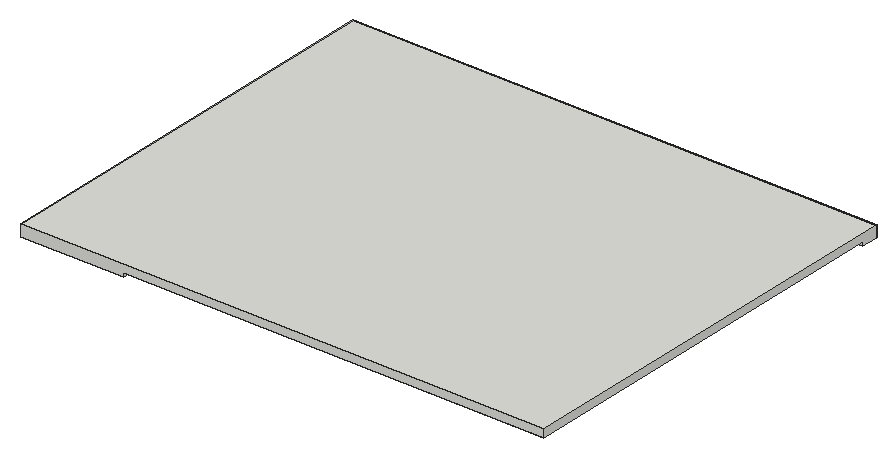
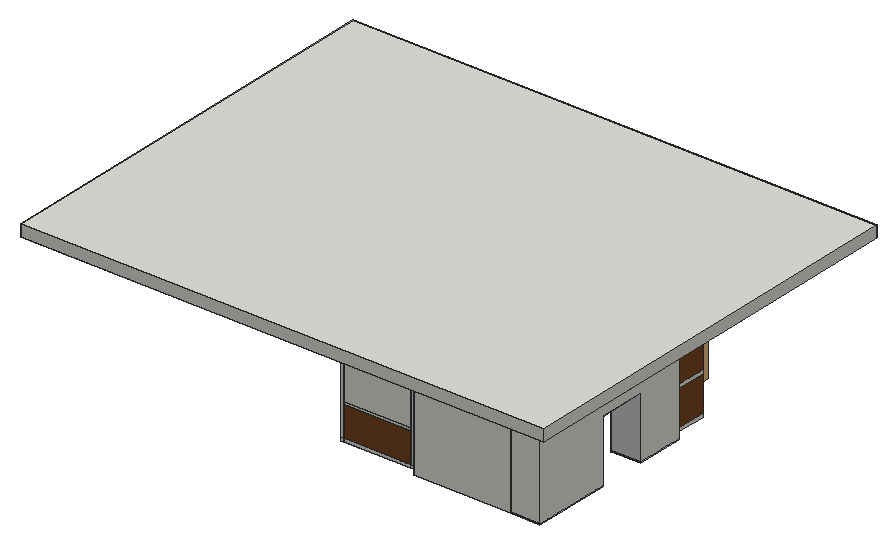
# SketchUp Ruby script. Lengths in inches.
U = 1.inch
M = Sketchup.active_model
def pt(a) = Geom::Point3d.new(a.map { |v| v * U })
def face(e, loops, mat)
  f = e.add_face(loops[0].map { |a| pt(a) })
  loops[1..].each { |l| e.add_face(l.map { |a| pt(a) }).erase! }
  f.material = f.back_material = mat if mat
  f
end
# faces: each face lists its corners as indices into pts; further lists are holes
def faces(e, pts, list, mat = nil) = list.each { |f| face(e, (f[0].is_a?(Array) ? f : [f]).map { |l| l.map { |i| pts[i] } }, mat) }
# xy, xz, yz: faces in a plane at the given z, y or x. An outline is a flat list of corners, or four numbers for a rectangle; further outlines are holes
def ring(l) = l.size == 4 ? [[l[0], l[1]], [l[2], l[1]], [l[2], l[3]], [l[0], l[3]]] : l.each_slice(2).to_a
def flat(e, list, mat, &to3) = list.each { |f| face(e, (f[0].is_a?(Array) ? f : [f]).map { |l| ring(l).map { |u, v| to3.(u, v) } }, mat) }
def xy(e, z, list, mat = nil) = flat(e, list, mat) { |x, y| [x, y, z] }
def xz(e, y, list, mat = nil) = flat(e, list, mat) { |x, z| [x, y, z] }
def yz(e, x, list, mat = nil) = flat(e, list, mat) { |y, z| [x, y, z] }
def lines(e, pts, list) = list.each { |a, b| e.add_line(pt(pts[a]), pt(pts[b])) }
# prism: a flat outline (further loops are holes) pulled along v
def prism(e, loops, v, mat = nil)
  f = face(e, loops, mat); d = Geom::Vector3d.new(v.map { |x| x * U })
  f.pushpull(f.normal.samedirection?(d) ? d.length : -d.length)
end
def box(e, o, s, mat = nil) = prism(e, [[o, [o[0] + s[0], o[1], o[2]], [o[0] + s[0], o[1] + s[1], o[2]], [o[0], o[1] + s[1], o[2]]]], [0, 0, s[2]], mat)
def at(x, y, z, deg = 0) = Geom::Transformation.translation(pt([x, y, z])) * Geom::Transformation.rotation(ORIGIN, Z_AXIS, deg.degrees)
def axes(o, x, y, z) = Geom::Transformation.new([*x, 0, *y, 0, *z, 0, *pt(o).to_a, 1])
def part(name) = M.definitions.add(name)
# library, detail: a bought-in or finely detailed component or shape, given as its bounding box
def library(name, o, s) = part(name).tap { |d| box(d.entities, o, s) }
def detail(e, o, s) = box(e.add_group.entities, o, s)
def put(e, d, t, mat = nil) = e.add_instance(d, t).tap { |i| i.material = mat if mat }
def group(e, t, mat = nil) = e.add_group.tap { |g| g.transformation = t; g.material = mat if mat }.entities
root = M.entities
M.materials.add("Emissive").color = [223, 228, 179]
M.materials.add("Generic").color = [71, 77, 71]
M.materials.add("Generic\#1").color = [198, 203, 199]
M.materials.add("Gold 10k").color = [251, 232, 180]
M.materials.add("[Wood Floor Light]").color = [204, 176, 127]
M.materials.add("[Wood Veneer 01]").color = [120, 70, 37]
c1 = library("kitchen utensils",[-21.58,227.67,74.34],[25.67,8.97,31.25])
c2 = library("Tlon Light 1950 Ceiling 152 010",[-38.39,-38.39,-3.78],[76.78,76.78,3.41])
c3 = library("Microwave 116-11",[-7.27,-5.23,0],[14.54,10.46,7.87])
c4 = library("Potted Plant 50-23",[-3.4,-3.5,0],[6.8,7,9.93])
c5 = library("Pendant 02 114-03",[-6.79,-6.8,-58.42],[13.6,13.6,58.44])
c6 = library("Peperomia 450 001",[-6.6875,-10.1875,-9.42],[16.7,12.74,19.03])
xy(root,72.9375,[[9,120.99,24.25,146.7],[9,172.41,24.25,172.41,24.25,198.875,25,198.875,25,214.125,9,214.125],[25,198.875,76.5,214.125]])
xy(root,72.9375,[[24.25,120.99,25,146.7],[24.25,172.41,25,198.125],[24.25,198.125,76.5,198.875]],"Gold 10k")
xy(root,73.34,[[9,120.99,24.25,146.7],[9,172.41,24.25,172.41,24.25,198.875,25,198.875,25,214.125,9,214.125]])
xy(root,73.34,[[24.25,120.99,25,133.84],[24.25,134.24,25,146.7],[24.25,172.41,25,185.27],[24.25,185.67,25,198.125],[24.25,198.125,25,198.875],
  [25,198.125,42.17,198.875],[42.57,198.125,59.33,198.875],[59.73,198.125,76.5,198.875]],"Gold 10k")
xy(root,74.34,[[43.57,198.125,58.33,210.125],[60.73,198.125,75.5,210.125]],"[Wood Floor Light]")
xy(root,75.04,[[10.8125,103.125,10.8125,119.26,25,119.26,25,107.5625,24.96,106.98,24.85,106.41,24.66,105.86,24.41,105.34,24.08,104.86,23.7,104.42,23.26,104.04,22.78,103.72,22.26,103.46,21.71,103.28,21.14,103.16,20.5625,103.125]],"[Wood Veneer 01]")
xy(root,75.875,[[78.25,188.8125,114.125,214.125]],"[Wood Veneer 01]")
xy(root,76.74,[[10.8125,103.125,20.5625,103.125,21.14,103.16,21.71,103.28,22.26,103.46,22.78,103.72,23.26,104.04,23.7,104.42,24.08,104.86,24.41,105.34,24.66,105.86,24.85,106.41,24.96,106.98,25,107.5625,25,119.26,10.8125,119.26]],"[Wood Veneer 01]")
xy(root,77.5,[[78.25,188.8125,114.125,214.125]],"[Wood Veneer 01]")
xy(root,85.24,[[43.57,208.125,58.33,210.125],[60.73,208.125,75.5,210.125]],"Emissive")
xy(root,85.24,[[43.57,198.3125,58.33,208.125],[60.73,198.3125,75.5,208.125]],"[Wood Floor Light]")
xy(root,86.49,[[43.57,198.3125,58.33,210.125],[60.73,198.3125,75.5,210.125]],"[Wood Floor Light]")
xy(root,93.85,[[78.25,212.125,114.125,214.125]],"Emissive")
xy(root,93.85,[[78.25,188.8125,114.125,212.125]],"[Wood Veneer 01]")
xy(root,94.92,[[78.25,188.8125,114.125,189.5625]],"Gold 10k")
xy(root,95.32,[[78.65,188.8125,95.79,189.5625],[96.1875,188.8125,113.73,189.5625]],"Gold 10k")
xy(root,96.04,[[10.8125,103.125,10.8125,119.26,25,119.26,25,107.5625,24.96,106.98,24.85,106.41,24.66,105.86,24.41,105.34,24.08,104.86,23.7,104.42,23.26,104.04,22.78,103.72,22.26,103.46,21.71,103.28,21.14,103.16,20.5625,103.125]],"[Wood Veneer 01]")
xy(root,96.68,[[43.57,208.125,58.33,210.125],[60.73,208.125,75.5,210.125]],"Emissive")
xy(root,96.68,[[43.57,198.3125,58.33,208.125],[60.73,198.3125,75.5,208.125]],"[Wood Floor Light]")
xy(root,97.74,[[10.8125,103.125,20.5625,103.125,21.14,103.16,21.71,103.28,22.26,103.46,22.78,103.72,23.26,104.04,23.7,104.42,24.08,104.86,24.41,105.34,24.66,105.86,24.85,106.41,24.96,106.98,25,107.5625,25,119.26,10.8125,119.26]],"[Wood Veneer 01]")
xy(root,97.93,[[43.57,198.3125,58.33,210.125],[60.73,198.3125,75.5,210.125]],"[Wood Floor Light]")
xy(root,106.4375,[[9,146.7,25,172.41]],"[Wood Veneer 01]")
xy(root,106.8125,[[9,146.7,24.25,172.41]])
xy(root,106.8125,[[24.25,146.7,25,172.41]],"Gold 10k")
xy(root,107.21,[[24.25,146.7,25,159.56],[24.25,159.96,25,172.41]],"Gold 10k")
xy(root,108.03,[[43.57,208.125,58.33,210.125],[60.73,208.125,75.5,210.125]],"Emissive")
xy(root,108.03,[[43.57,198.125,58.33,208.125],[60.73,198.125,75.5,208.125]],"[Wood Floor Light]")
xy(root,109.03,[[42.57,198.125,59.33,198.875],[59.73,198.125,76.5,198.875]],"Gold 10k")
xy(root,109.43,[[42.57,198.125,59.33,198.875],[59.73,198.125,76.5,198.875]],"Gold 10k")
xy(root,114.48,[[10.8125,119.26,13.21,119.92]])
xy(root,114.48,[[13.21,103.125,13.21,119.26,25,119.26,25,120.99,55.3125,120.99,55.3125,103.125]],"[Wood Veneer 01]")
xy(root,118.1,[[78.65,188.8125,95.79,189.5625],[96.1875,188.8125,113.73,189.5625]],"Gold 10k")
xy(root,118.5,[[114.125,188.8125,115.875,214.125],[78.25,189.5625,114.125,214.125]])
xy(root,118.5,[[78.25,188.8125,114.125,189.5625]],"Gold 10k")
xy(root,119.1875,[[9,120.99,9,214.125,25,214.125,25,198.125,24.25,198.125,24.25,120.99],[24.25,172.41,25,185.27],[42.57,198.125,59.33,198.875],[59.73,198.125,76.5,198.875],[25,198.875,76.5,214.125]])
xy(root,119.1875,[[24.25,120.99,25,133.84],[24.25,134.24,25,146.7],[24.25,146.7,25,159.56],[24.25,159.96,25,172.41],[24.25,185.67,25,198.125],
  [25,198.125,42.17,198.875]],"Gold 10k")
xy(root,119.4375,[[9,120.99,9,214.125,25,214.125,25,198.125,24.25,198.125,24.25,120.99],[25,198.875,76.5,214.125]])
xy(root,119.4375,[[24.25,120.99,25,198.125],[25,198.125,76.5,198.875]],"Gold 10k")
xy(root,120,[[0,0,9,223.125],[9,0,55.3125,103.125],[9,103.125,55.3125,120.99],[9,120.99,25,214.125],[76.5,188.8125,78.25,214.125],
  [78.25,188.8125,114.125,190.125],[114.125,188.8125,115.875,214.125],[78.25,190.125,114.125,214.125],[78.25,190.125,114.125,214.125],[25,198.125,76.5,214.125],
  [9,214.125,280.625,223.125]])
xy(root,120,[[[55.3125,103.125,55.3125,120.99,25,120.99,25,198.125,76.5,198.125,76.5,188.8125,115.875,188.8125,115.875,214.125,120,214.125,120,103.125],[62.86,110.67,112.45,110.67,112.45,181.27,68.95,181.27,68.95,190.58,32.55,190.58,32.55,128.53,62.86,128.53]],[48.41,135.56,48.41,176.5,55.1,176.5,55.1,140.62,103.28,140.62,103.28,135.56],[[64.44,146.92,76.63,163.8],[68.11,152.46,72.97,158.13]]],"[Wood Veneer 01]")
xy(root,122,[[55.3125,0,280.625,103.125],[[55.3125,103.125,120,103.125,120,214.125,115.875,214.125,115.875,188.8125,76.5,188.8125,76.5,198.125,25,198.125,25,120.99,55.3125,120.99],[60.86,108.67,60.86,126.53,30.55,126.53,30.55,192.58,70.95,192.58,70.95,183.27,114.45,183.27,114.45,108.67]],[120,103.125,280.625,214.125],[50.41,137.56,103.28,137.56,103.28,138.62,53.1,138.62,53.1,176.5,50.41,176.5],[[64.44,148.92,74.63,161.8],[66.11,150.46,72.97,158.13]]])
xy(root,122,[[60.86,108.67,62.86,128.53],[62.86,108.67,112.45,110.67],[112.45,108.67,114.45,181.27],[30.55,126.53,32.55,190.58],[32.55,126.53,60.86,128.53],
  [48.41,135.56,50.41,176.5],[50.41,135.56,55.1,137.56],[55.1,135.56,103.28,137.56],[53.1,138.62,55.1,176.5],[55.1,138.62,103.28,140.62],
  [64.44,146.92,74.63,148.92],[74.63,146.92,76.63,163.8],[66.11,150.46,72.97,152.46],[66.11,152.46,68.11,158.13],[64.44,161.8,74.63,163.8],
  [68.95,181.27,78.25,183.27],[78.25,181.27,114.45,183.27],[68.95,183.27,70.95,190.58],[30.55,190.58,70.95,192.58]],"Emissive")
xy(root,124,[[[60.86,108.67,60.86,126.53,30.55,126.53,30.55,192.58,70.95,192.58,70.95,183.27,114.45,183.27,114.45,108.67],[50.41,137.56,103.28,137.56,103.28,138.62,53.1,138.62,53.1,176.5,50.41,176.5],[64.44,148.92,74.63,161.8]],[66.11,150.46,72.97,158.13]])
xy(root,126,[[0,0,280.625,223.125]])
xz(root,0,[[0,120,55.3125,120,55.3125,122,280.625,122,280.625,126,0,126]])
xz(root,103.125,[[55.3125,120,120,122]])
xz(root,103.125,[[10.8125,75.04,20.5625,76.74],[10.8125,96.04,20.5625,97.74]],"[Wood Veneer 01]")
xz(root,108.67,[[60.86,122,114.45,124]],"Emissive")
xz(root,110.67,[[62.86,120,112.45,122]])
xz(root,119.26,[[10.8125,75.04,25,76.74],[10.8125,96.04,25,97.74]])
xz(root,119.26,[[10.8125,76.74,25,96.04],[10.8125,97.74,25,114.48]],"[Wood Veneer 01]")
xz(root,119.92,[[10.8125,112.09,10.8125,114.48,13.21,114.48,12.89,114.46,12.59,114.4,12.29,114.3,12.01,114.16,11.75,113.99,11.51,113.78,11.31,113.55,11.13,113.29,10.99,113,10.89,112.71,10.83,112.4]])
xz(root,120.99,[[9,72.9375,24.25,73.34],[24.25,72.9375,25,73.34],[9,73.34,25,119.1875],[9,119.1875,24.25,119.4375],[9,119.4375,25,120],
  [25,120,55.3125,122]])
xz(root,120.99,[[25,114.48,25,119.1875,24.25,119.1875,24.25,119.4375,25,119.4375,25,120,55.3125,120,55.3125,114.48]],"[Wood Veneer 01]")
xz(root,126.53,[[30.55,122,60.86,124]],"Emissive")
xz(root,128.53,[[32.55,120,62.86,122]],"[Wood Veneer 01]")
xz(root,133.84,[[24.25,73.34,25,119.1875]],"Gold 10k")
xz(root,134.24,[[24.25,73.34,25,119.1875]],"Gold 10k")
xz(root,135.56,[[48.41,120,55.1,122],[55.1,120,103.28,122]],"[Wood Veneer 01]")
xz(root,137.56,[[50.41,122,55.1,124],[55.1,122,103.28,124]],"Emissive")
xz(root,138.62,[[53.1,122,103.28,124]],"Emissive")
xz(root,140.62,[[55.1,120,103.28,122]],"[Wood Veneer 01]")
xz(root,146.7,[[9,72.9375,24.25,73.34],[9,106.4375,25,106.8125],[24.25,106.8125,25,107.21]])
xz(root,146.7,[[9,73.34,25,106.4375]],"Generic\#1")
xz(root,146.92,[[64.44,120,76.63,122]],"[Wood Veneer 01]")
xz(root,148.92,[[64.44,122,74.63,124]],"Emissive")
xz(root,150.46,[[66.11,122,72.97,124]],"Emissive")
xz(root,152.46,[[68.11,120,72.97,122]])
xz(root,158.13,[[68.11,120,72.97,122]])
xz(root,158.13,[[66.11,122,72.97,124]],"Emissive")
xz(root,159.56,[[24.25,107.21,25,119.1875]],"Gold 10k")
xz(root,159.96,[[24.25,107.21,25,119.1875]],"Gold 10k")
xz(root,161.8,[[64.44,122,74.63,124]],"Emissive")
xz(root,163.8,[[64.44,120,76.63,122]])
xz(root,172.41,[[9,106.4375,25,106.8125],[24.25,106.8125,25,107.21]])
xz(root,172.41,[[9,72.9375,24.25,73.34]],"Generic\#1")
xz(root,172.41,[[9,73.34,25,106.4375]],"[Wood Veneer 01]")
xz(root,176.5,[[48.41,120,55.1,122],[50.41,122,53.1,124]])
xz(root,181.27,[[68.95,120,78.25,122],[78.25,120,112.45,122]],"[Wood Veneer 01]")
xz(root,183.27,[[70.95,122,78.25,124],[78.25,122,114.45,124]],"Emissive")
xz(root,185.27,[[24.25,73.34,25,119.1875]],"Gold 10k")
xz(root,185.67,[[24.25,73.34,25,119.1875]],"Gold 10k")
xz(root,188.8125,[[76.5,120,78.25,122],[78.25,120,114.125,122],[114.125,120,115.875,122]])
xz(root,188.8125,[[78.65,95.32,95.79,118.1],[96.1875,95.32,113.73,118.1]],"Generic\#1")
xz(root,188.8125,[[78.25,75.875,114.125,77.5],[78.25,93.85,114.125,94.92],[78.25,118.5,114.125,120],[114.125,118.5,115.875,120]],"[Wood Veneer 01]")
xz(root,189.5625,[[[78.25,94.92,114.125,118.5],[78.65,95.32,113.73,118.1]],[95.79,95.32,96.1875,118.1]],"Gold 10k")
xz(root,190.58,[[32.55,120,68.95,122]],"[Wood Veneer 01]")
xz(root,192.58,[[30.55,122,70.95,124]],"Emissive")
xz(root,198.125,[[25,120,76.5,122]])
xz(root,198.125,[[25,73.34,42.17,119.1875]],"Generic")
xz(root,198.125,[[42.57,109.43,59.33,119.1875],[59.73,109.43,76.5,119.1875],[25,119.4375,76.5,120]],"Generic\#1")
xz(root,198.125,[[24.25,119.1875,25,119.4375]],"Gold 10k")
xz(root,198.125,[[[42.57,73.34,59.33,109.03],[43.57,74.34,58.33,108.03]],[[59.73,73.34,76.5,109.03],[60.73,74.34,75.5,108.03]]],"[Wood Floor Light]")
xz(root,198.3125,[[43.57,85.24,58.33,86.49],[60.73,85.24,75.5,86.49],[43.57,96.68,58.33,97.93],[60.73,96.68,75.5,97.93]],"[Wood Floor Light]")
xz(root,198.875,[[24.25,72.9375,25,73.34],[25,72.9375,76.5,73.34],[42.17,73.34,42.57,119.1875],[59.33,73.34,59.73,119.1875],[42.57,109.03,59.33,109.43],
  [59.73,109.03,76.5,109.43],[25,119.1875,76.5,119.4375]],"Gold 10k")
xz(root,210.125,[[43.57,85.24,58.33,86.49],[60.73,85.24,75.5,86.49],[43.57,96.68,58.33,97.93],[60.73,96.68,75.5,97.93]])
xz(root,210.125,[[43.57,74.34,58.33,85.24],[60.73,74.34,75.5,85.24],[43.57,86.49,58.33,96.68],[60.73,86.49,75.5,96.68],[43.57,97.93,58.33,108.03],
  [60.73,97.93,75.5,108.03]],"[Wood Floor Light]")
xz(root,214.125,[[9,72.9375,25,73.34],[25,72.9375,76.5,119.1875],[9,73.34,25,119.1875],[76.5,75.875,78.25,77.5],[78.25,75.875,114.125,77.5],
  [114.125,75.875,115.875,77.5],[76.5,77.5,78.25,120],[114.125,77.5,115.875,118.5],[78.25,93.85,114.125,94.92],[78.25,94.92,114.125,118.5],
  [78.25,118.5,114.125,120],[114.125,118.5,115.875,120],[9,119.1875,25,119.4375],[25,119.1875,76.5,119.4375],[9,119.4375,25,120],
  [25,119.4375,76.5,120],[115.875,120,120,122],[120,120,280.625,122]])
xz(root,214.125,[[78.25,77.5,114.125,93.85]],"[Wood Veneer 01]")
xz(root,223.125,[[0,120,280.625,126]])
yz(root,0,[[0,120,223.125,126]])
yz(root,9,[[120.99,72.9375,146.7,73.34],[172.41,72.9375,214.125,73.34],[120.99,73.34,120.99,119.1875,214.125,119.1875,214.125,73.34,172.41,73.34,172.41,106.8125,146.7,106.8125,146.7,73.34],[146.7,106.4375,172.41,106.8125],[120.99,119.1875,214.125,119.4375],
  [120.99,119.4375,214.125,120]])
yz(root,10.8125,[[103.125,75.04,119.26,76.74],[103.125,96.04,119.26,97.74],[119.26,112.09,119.92,114.48]])
yz(root,10.8125,[[103.125,76.74,119.26,96.04],[103.125,97.74,119.26,112.09]],"[Wood Veneer 01]")
yz(root,24.25,[[120.99,72.9375,146.7,73.34],[172.41,72.9375,198.875,73.34],[133.84,73.34,134.24,119.1875],[185.27,73.34,185.67,119.1875],[146.7,106.8125,172.41,107.21],
  [159.56,107.21,159.96,119.1875],[120.99,119.1875,198.125,119.4375]],"Gold 10k")
yz(root,25,[[198.875,72.9375,214.125,73.34],[198.125,73.34,214.125,119.1875],[146.7,106.4375,172.41,106.8125],[198.875,119.1875,214.125,119.4375],[198.125,119.4375,214.125,120],
  [120.99,120,198.125,122]])
yz(root,25,[[146.7,107.21,159.56,119.1875],[159.96,107.21,172.41,119.1875]],"Generic")
yz(root,25,[[120.99,73.34,133.84,119.1875],[134.24,73.34,146.7,119.1875],[172.41,73.34,185.27,119.1875],[185.67,73.34,198.125,119.1875],[120.99,119.4375,198.125,120]],"Generic\#1")
yz(root,25,[[198.125,119.1875,198.875,119.4375]],"Gold 10k")
yz(root,25,[[107.5625,75.04,119.26,76.74],[107.5625,96.04,119.26,97.74]],"[Wood Veneer 01]")
yz(root,30.55,[[126.53,122,192.58,124]],"Emissive")
yz(root,32.55,[[128.53,120,190.58,122]],"[Wood Veneer 01]")
yz(root,42.17,[[198.125,73.34,198.875,119.1875]],"Gold 10k")
yz(root,42.57,[[198.125,109.43,198.875,119.1875]])
yz(root,42.57,[[198.125,73.34,198.875,109.03]],"Gold 10k")
yz(root,43.57,[[198.3125,85.24,210.125,86.49],[198.3125,96.68,210.125,97.93]])
yz(root,43.57,[[198.125,74.34,210.125,74.34,210.125,85.24,198.3125,85.24,198.3125,86.49,210.125,86.49,210.125,96.68,198.3125,96.68,198.3125,97.93,210.125,97.93,210.125,108.03,198.125,108.03]],"[Wood Floor Light]")
yz(root,48.41,[[135.56,120,176.5,122]])
yz(root,50.41,[[137.56,122,176.5,124]],"Emissive")
yz(root,53.1,[[138.62,122,176.5,124]],"Emissive")
yz(root,55.1,[[140.62,120,176.5,122]],"[Wood Veneer 01]")
yz(root,55.3125,[[0,120,103.125,122],[103.125,120,120.99,122]])
yz(root,55.3125,[[103.125,114.48,120.99,120]],"[Wood Veneer 01]")
yz(root,58.33,[[198.3125,85.24,210.125,86.49],[198.3125,96.68,210.125,97.93]])
yz(root,58.33,[[198.125,74.34,198.125,108.03,210.125,108.03,210.125,97.93,198.3125,97.93,198.3125,96.68,210.125,96.68,210.125,86.49,198.3125,86.49,198.3125,85.24,210.125,85.24,210.125,74.34]],"[Wood Floor Light]")
yz(root,59.33,[[198.125,73.34,198.875,109.03],[198.125,109.43,198.875,119.1875]],"Gold 10k")
yz(root,59.73,[[198.125,73.34,198.875,109.03],[198.125,109.43,198.875,119.1875]],"Gold 10k")
yz(root,60.73,[[198.3125,85.24,210.125,86.49],[198.3125,96.68,210.125,97.93]])
yz(root,60.73,[[198.125,74.34,210.125,74.34,210.125,85.24,198.3125,85.24,198.3125,86.49,210.125,86.49,210.125,96.68,198.3125,96.68,198.3125,97.93,210.125,97.93,210.125,108.03,198.125,108.03]],"[Wood Floor Light]")
yz(root,60.86,[[108.67,122,126.53,124]],"Emissive")
yz(root,62.86,[[110.67,120,128.53,122]],"[Wood Veneer 01]")
yz(root,64.44,[[146.92,120,163.8,122]])
yz(root,64.44,[[148.92,122,161.8,124]],"Emissive")
yz(root,66.11,[[150.46,122,158.13,124]],"Emissive")
yz(root,68.11,[[152.46,120,158.13,122]])
yz(root,68.95,[[181.27,120,190.58,122]])
yz(root,70.95,[[183.27,122,192.58,124]],"Emissive")
yz(root,72.97,[[152.46,120,158.13,122]])
yz(root,72.97,[[150.46,122,158.13,124]],"Emissive")
yz(root,74.63,[[148.92,122,161.8,124]],"Emissive")
yz(root,75.5,[[198.3125,85.24,210.125,86.49],[198.3125,96.68,210.125,97.93]])
yz(root,75.5,[[198.125,74.34,198.125,108.03,210.125,108.03,210.125,97.93,198.3125,97.93,198.3125,96.68,210.125,96.68,210.125,86.49,198.3125,86.49,198.3125,85.24,210.125,85.24,210.125,74.34]],"[Wood Floor Light]")
yz(root,76.5,[[198.875,72.9375,214.125,72.9375,214.125,75.875,198.125,75.875,198.125,73.34,198.875,73.34],[198.125,75.875,214.125,77.5],[198.125,77.5,214.125,77.5,214.125,119.1875,198.125,119.1875,198.125,109.43,198.875,109.43,198.875,109.03,198.125,109.03],[198.875,119.1875,214.125,119.4375],[198.125,119.4375,214.125,120],
  [188.8125,120,198.125,122]])
yz(root,76.63,[[146.92,120,163.8,122]],"[Wood Veneer 01]")
yz(root,78.25,[[188.8125,93.85,190.125,94.92],[190.125,93.85,214.125,94.92],[189.5625,94.92,190.125,118.5],[190.125,94.92,214.125,118.5]])
yz(root,78.25,[[188.8125,94.92,189.5625,118.5]],"Gold 10k")
yz(root,78.25,[[188.8125,77.5,214.125,93.85]],"[Wood Veneer 01]")
yz(root,78.65,[[188.8125,95.32,189.5625,118.1]],"Gold 10k")
yz(root,95.79,[[188.8125,95.32,189.5625,118.1]],"Gold 10k")
yz(root,96.1875,[[188.8125,95.32,189.5625,118.1]],"Gold 10k")
yz(root,103.28,[[137.56,122,138.62,124]])
yz(root,103.28,[[135.56,120,140.62,122]],"[Wood Veneer 01]")
yz(root,112.45,[[110.67,120,181.27,122]])
yz(root,113.73,[[188.8125,95.32,189.5625,118.1]],"Gold 10k")
yz(root,114.125,[[188.8125,75.875,190.125,77.5],[190.125,75.875,214.125,77.5],[188.8125,93.85,190.125,94.92],[190.125,93.85,214.125,94.92],[189.5625,94.92,190.125,118.5],
  [190.125,94.92,214.125,118.5],[188.8125,118.5,190.125,120],[190.125,118.5,214.125,120]])
yz(root,114.125,[[188.8125,94.92,189.5625,118.5]],"Gold 10k")
yz(root,114.125,[[188.8125,77.5,214.125,93.85]],"[Wood Veneer 01]")
yz(root,114.45,[[108.67,122,183.27,124]],"Emissive")
yz(root,115.875,[[188.8125,120,214.125,122]])
yz(root,115.875,[[188.8125,118.5,214.125,120]],"[Wood Veneer 01]")
yz(root,120,[[103.125,120,214.125,122]])
yz(root,280.625,[[214.125,120,223.125,120,223.125,126,0,126,0,122,214.125,122]])
p = [[21.14,103.16,76.74],[20.5625,103.125,76.74],[20.5625,103.125,75.04],[21.14,103.16,75.04],[21.71,103.28,76.74],[21.71,103.28,75.04],
  [22.26,103.46,76.74],[22.26,103.46,75.04],[22.78,103.72,76.74],[22.78,103.72,75.04],[23.26,104.04,76.74],[23.26,104.04,75.04],
  [23.7,104.42,76.74],[23.7,104.42,75.04],[24.08,104.86,76.74],[24.08,104.86,75.04],[24.41,105.34,76.74],[24.41,105.34,75.04],
  [24.66,105.86,76.74],[24.66,105.86,75.04],[24.85,106.41,76.74],[24.85,106.41,75.04],[24.96,106.98,76.74],[24.96,106.98,75.04],
  [25,107.5625,76.74],[25,107.5625,75.04],[21.14,103.16,97.74],[20.5625,103.125,97.74],[20.5625,103.125,96.04],[21.14,103.16,96.04],
  [21.71,103.28,97.74],[21.71,103.28,96.04],[22.26,103.46,97.74],[22.26,103.46,96.04],[22.78,103.72,97.74],[22.78,103.72,96.04],
  [23.26,104.04,97.74],[23.26,104.04,96.04],[23.7,104.42,97.74],[23.7,104.42,96.04],[24.08,104.86,97.74],[24.08,104.86,96.04],
  [24.41,105.34,97.74],[24.41,105.34,96.04],[24.66,105.86,97.74],[24.66,105.86,96.04],[24.85,106.41,97.74],[24.85,106.41,96.04],
  [24.96,106.98,97.74],[24.96,106.98,96.04],[25,107.5625,97.74],[25,107.5625,96.04],[10.83,103.125,112.4],[10.8125,103.125,112.09],
  [10.8125,119.26,112.09],[10.8125,119.92,112.09],[10.83,119.92,112.4],[10.89,103.125,112.71],[10.89,119.92,112.71],[10.99,103.125,113],
  [10.99,119.92,113],[11.13,103.125,113.29],[11.13,119.92,113.29],[11.31,103.125,113.55],[11.31,119.92,113.55],[11.51,103.125,113.78],
  [11.51,119.92,113.78],[11.75,103.125,113.99],[11.75,119.92,113.99],[12.01,103.125,114.16],[12.01,119.92,114.16],[12.29,103.125,114.3],
  [12.29,119.92,114.3],[12.59,103.125,114.4],[12.59,119.92,114.4],[12.89,103.125,114.46],[12.89,119.92,114.46],[13.21,103.125,114.48],
  [13.21,119.92,114.48],[13.21,119.26,114.48],[78.25,190.125,75.875],[78.25,190.125,77.5],[78.25,190.125,118.5],[78.25,190.125,120],
  [10.8125,103.125,114.48],[10.8125,119.26,114.48]]
faces(root,p,[[0,1,2,3],[4,0,3,5],[6,4,5,7],[8,6,7,9],[10,8,9,11],[12,10,11,13],[14,12,13,15],[16,14,15,17],
  [18,16,17,19],[20,18,19,21],[22,20,21,23],[24,22,23,25],[26,27,28,29],[30,26,29,31],[32,30,31,33],[34,32,33,35],
  [36,34,35,37],[38,36,37,39],[40,38,39,41],[42,40,41,43],[44,42,43,45],[46,44,45,47],[48,46,47,49],[50,48,49,51],
  [52,53,54,55,56],[57,52,56,58],[59,57,58,60],[61,59,60,62],[63,61,62,64],[65,63,64,66],[67,65,66,68],[69,67,68,70],
  [71,69,70,72],[73,71,72,74],[75,73,74,76],[77,75,76,78,79]],"[Wood Veneer 01]")
lines(root,p,[[80,81],[82,83],[84,85]])
put(root,c1,at(68.18,-28.25,0))
put(root,c2,axes([18.1,109.0625,75.13],[0.0252,0,0],[0,0.0252,0],[0,0,0.0252]))
put(root,c3,axes([100.49,197.46,77.5],[1.65,0,0],[0,1.4,0],[0,0,1.31]))
put(root,c4,axes([83.65,195.75,77.5],[1.45686,0,0],[0,1.42,0],[0,0,1.27]))
put(root,c5,axes([35.25,106.93,114.49],[1,0,0],[0,1,0],[0,0,0.58]))
put(root,c5,axes([50.31,106.93,114.49],[1,0,0],[0,1,0],[0,0,0.58]))
put(root,c6,axes([22.41,107.92,99.25],[1.12,0,0],[0,1.3447,0],[0,0,1.16]))
put(root,c2,axes([18.1,109.47,96.13],[0.0252,0,0],[0,0.0252,0],[0,0,0.0252]))
put(root,c2,axes([18.1,109.0625,114.58],[0.0252,0,0],[0,0.0252,0],[0,0,0.0252]))
put(root,c2,axes([104.94,183.68,120.08],[0.0252,0,0],[0,0.0252,0],[0,0,0.0252]))
put(root,c2,axes([85.25,183.68,120.08],[0.0252,0,0],[0,0.0252,0],[0,0,0.0252]))
put(root,c2,axes([73,183.68,120.08],[0.0252,0,0],[0,0.0252,0],[0,0,0.0252]))
put(root,c2,axes([73,193.43,120.08],[0.0252,0,0],[0,0.0252,0],[0,0,0.0252]))
put(root,c2,axes([56.69,193.43,120.08],[0.0252,0,0],[0,0.0252,0],[0,0,0.0252]))
put(root,c2,axes([36.06,193.43,120.08],[0.0252,0,0],[0,0.0252,0],[0,0,0.0252]))
put(root,c2,axes([28.06,193.43,120.08],[0.0252,0,0],[0,0.0252,0],[0,0,0.0252]))
put(root,c2,axes([28.06,173.81,120.08],[0.0252,0,0],[0,0.0252,0],[0,0,0.0252]))
put(root,c2,axes([28.06,145.74,120.08],[0.0252,0,0],[0,0.0252,0],[0,0,0.0252]))
